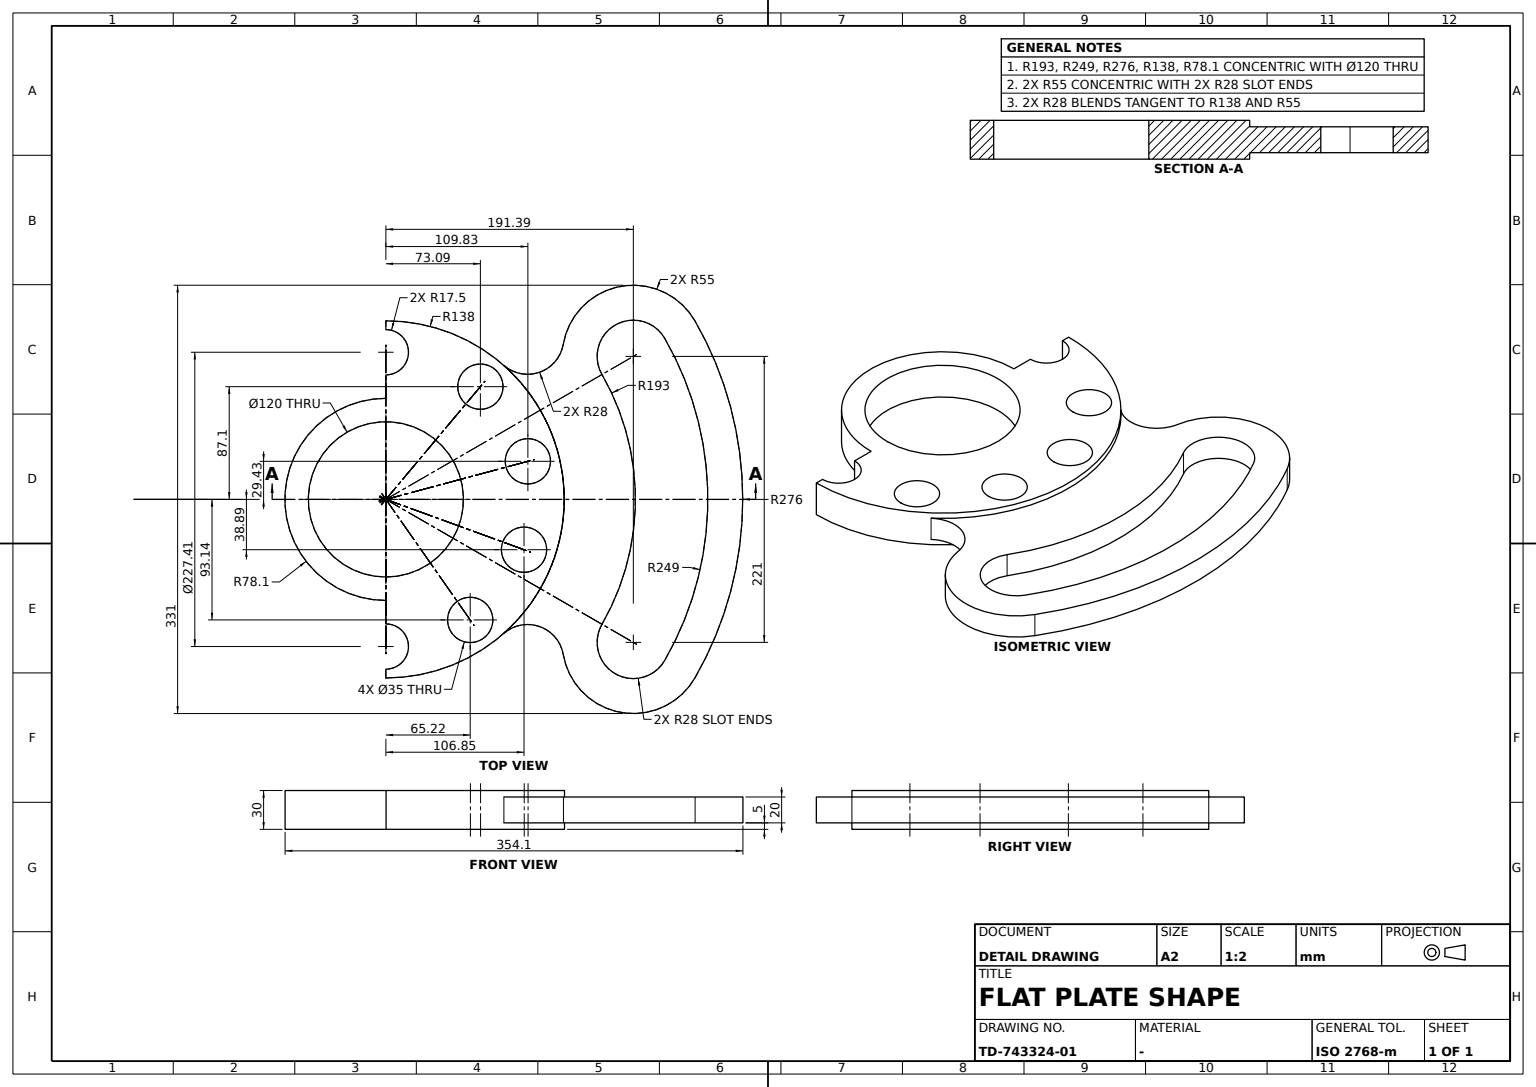
ISO-10303-21;
HEADER;
FILE_DESCRIPTION((''),'2;1');
FILE_NAME('','',(''),(''),'','','');
FILE_SCHEMA(('AUTOMOTIVE_DESIGN'));
ENDSEC;
DATA;
#1=APPLICATION_CONTEXT('');
#2=PRODUCT_CONTEXT('',#1,'mechanical');
#3=PRODUCT('','','',(#2));
#4=PRODUCT_DEFINITION_FORMATION('','',#3);
#5=PRODUCT_DEFINITION_CONTEXT('',#1,'design');
#6=PRODUCT_DEFINITION('','',#4,#5);
#7=PRODUCT_DEFINITION_SHAPE('','',#6);
#8=(LENGTH_UNIT()NAMED_UNIT(*)SI_UNIT(.MILLI.,.METRE.));
#9=(NAMED_UNIT(*)PLANE_ANGLE_UNIT()SI_UNIT($,.RADIAN.));
#10=(NAMED_UNIT(*)SI_UNIT($,.STERADIAN.)SOLID_ANGLE_UNIT());
#11=UNCERTAINTY_MEASURE_WITH_UNIT(LENGTH_MEASURE(0.005),#8,'distance_accuracy_value','');
#12=(GEOMETRIC_REPRESENTATION_CONTEXT(3)GLOBAL_UNCERTAINTY_ASSIGNED_CONTEXT((#11))GLOBAL_UNIT_ASSIGNED_CONTEXT((#8,#9,#10))REPRESENTATION_CONTEXT('',''));
#13=CARTESIAN_POINT('',(131.205128,0.,15.));
#14=VERTEX_POINT('',#13);
#15=CARTESIAN_POINT('',(138.,0.,15.));
#16=VERTEX_POINT('',#15);
#17=CARTESIAN_POINT('',(0.,0.,15.));
#18=DIRECTION('',(1.,0.,0.));
#19=VECTOR('',#18,1000.);
#20=LINE('',#17,#19);
#21=EDGE_CURVE('',#14,#16,#20,.T.);
#22=ORIENTED_EDGE('',*,*,#21,.F.);
#23=CARTESIAN_POINT('',(131.205128,0.,-15.));
#24=VERTEX_POINT('',#23);
#25=DIRECTION('',(0.,0.,1.));
#26=VECTOR('',#25,1000.);
#27=LINE('',#23,#26);
#28=EDGE_CURVE('',#24,#14,#27,.T.);
#29=ORIENTED_EDGE('',*,*,#28,.F.);
#30=CARTESIAN_POINT('',(138.,0.,-15.));
#31=VERTEX_POINT('',#30);
#32=CARTESIAN_POINT('',(0.,0.,-15.));
#33=LINE('',#32,#19);
#34=EDGE_CURVE('',#24,#31,#33,.T.);
#35=ORIENTED_EDGE('',*,*,#34,.T.);
#36=LINE('',#30,#26);
#37=EDGE_CURVE('',#31,#16,#36,.T.);
#38=ORIENTED_EDGE('',*,*,#37,.T.);
#39=EDGE_LOOP('',(#22,#29,#35,#38));
#40=FACE_BOUND('',#39,.T.);
#41=CARTESIAN_POINT('',(-138.,0.,0.));
#42=DIRECTION('',(0.,-1.,0.));
#43=AXIS2_PLACEMENT_3D('',#41,#42,#18);
#44=PLANE('',#43);
#45=ADVANCED_FACE('',(#40),#44,.T.);
#46=CARTESIAN_POINT('',(60.,0.,15.));
#47=VERTEX_POINT('',#46);
#48=AXIS2_PLACEMENT_3D('',#17,#25,#18);
#49=CIRCLE('',#48,60.);
#50=EDGE_CURVE('',#47,#47,#49,.T.);
#51=ORIENTED_EDGE('',*,*,#50,.T.);
#52=EDGE_LOOP('',(#51));
#53=FACE_BOUND('',#52,.T.);
#54=CARTESIAN_POINT('',(60.,0.,-15.));
#55=VERTEX_POINT('',#54);
#56=AXIS2_PLACEMENT_3D('',#32,#25,#18);
#57=CIRCLE('',#56,60.);
#58=EDGE_CURVE('',#55,#55,#57,.T.);
#59=ORIENTED_EDGE('',*,*,#58,.F.);
#60=EDGE_LOOP('',(#59));
#61=FACE_BOUND('',#60,.T.);
#62=CARTESIAN_POINT('',(0.,0.,9.34));
#63=AXIS2_PLACEMENT_3D('',#62,#25,#18);
#64=CYLINDRICAL_SURFACE('',#63,60.);
#65=ADVANCED_FACE('',(#53,#61),#64,.F.);
#66=CARTESIAN_POINT('',(56.389444,106.84787,15.));
#67=VERTEX_POINT('',#66);
#68=CARTESIAN_POINT('',(38.889444,106.84787,15.));
#69=AXIS2_PLACEMENT_3D('',#68,#25,#18);
#70=CIRCLE('',#69,17.5);
#71=EDGE_CURVE('',#67,#67,#70,.T.);
#72=ORIENTED_EDGE('',*,*,#71,.T.);
#73=EDGE_LOOP('',(#72));
#74=FACE_BOUND('',#73,.T.);
#75=CARTESIAN_POINT('',(56.389444,106.84787,-15.));
#76=VERTEX_POINT('',#75);
#77=CARTESIAN_POINT('',(38.889444,106.84787,-15.));
#78=AXIS2_PLACEMENT_3D('',#77,#25,#18);
#79=CIRCLE('',#78,17.5);
#80=EDGE_CURVE('',#76,#76,#79,.T.);
#81=ORIENTED_EDGE('',*,*,#80,.F.);
#82=EDGE_LOOP('',(#81));
#83=FACE_BOUND('',#82,.T.);
#84=CARTESIAN_POINT('',(38.889444,106.84787,9.34));
#85=AXIS2_PLACEMENT_3D('',#84,#25,#18);
#86=CYLINDRICAL_SURFACE('',#85,17.5);
#87=ADVANCED_FACE('',(#74,#83),#86,.F.);
#88=CARTESIAN_POINT('',(-78.102497,0.,-15.));
#89=VERTEX_POINT('',#88);
#90=CARTESIAN_POINT('',(-78.102497,0.,15.));
#91=VERTEX_POINT('',#90);
#92=LINE('',#88,#26);
#93=EDGE_CURVE('',#89,#91,#92,.T.);
#94=ORIENTED_EDGE('',*,*,#93,.F.);
#95=CARTESIAN_POINT('',(78.102497,0.,-15.));
#96=VERTEX_POINT('',#95);
#97=CIRCLE('',#56,78.102497);
#98=EDGE_CURVE('',#89,#96,#97,.T.);
#99=ORIENTED_EDGE('',*,*,#98,.T.);
#100=CARTESIAN_POINT('',(78.102497,0.,15.));
#101=VERTEX_POINT('',#100);
#102=LINE('',#95,#26);
#103=EDGE_CURVE('',#96,#101,#102,.T.);
#104=ORIENTED_EDGE('',*,*,#103,.T.);
#105=CIRCLE('',#48,78.102497);
#106=EDGE_CURVE('',#91,#101,#105,.T.);
#107=ORIENTED_EDGE('',*,*,#106,.F.);
#108=EDGE_LOOP('',(#94,#99,#104,#107));
#109=FACE_BOUND('',#108,.T.);
#110=CARTESIAN_POINT('',(0.,0.,0.));
#111=AXIS2_PLACEMENT_3D('',#110,#25,#18);
#112=CYLINDRICAL_SURFACE('',#111,78.102497);
#113=ADVANCED_FACE('',(#109),#112,.T.);
#114=CARTESIAN_POINT('',(96.205128,0.,15.));
#115=VERTEX_POINT('',#114);
#116=CARTESIAN_POINT('',(96.205128,0.,-15.));
#117=VERTEX_POINT('',#116);
#118=LINE('',#116,#26);
#119=EDGE_CURVE('',#115,#117,#118,.F.);
#120=ORIENTED_EDGE('',*,*,#119,.F.);
#121=EDGE_CURVE('',#101,#115,#20,.T.);
#122=ORIENTED_EDGE('',*,*,#121,.F.);
#123=ORIENTED_EDGE('',*,*,#103,.F.);
#124=EDGE_CURVE('',#96,#117,#33,.T.);
#125=ORIENTED_EDGE('',*,*,#124,.T.);
#126=EDGE_LOOP('',(#120,#122,#123,#125));
#127=FACE_BOUND('',#126,.T.);
#128=ADVANCED_FACE('',(#127),#44,.T.);
#129=CARTESIAN_POINT('',(124.5,215.640326,10.));
#130=VERTEX_POINT('',#129);
#131=CARTESIAN_POINT('',(-124.5,215.640326,10.));
#132=VERTEX_POINT('',#131);
#133=CARTESIAN_POINT('',(0.,0.,10.));
#134=AXIS2_PLACEMENT_3D('',#133,#25,#18);
#135=CIRCLE('',#134,249.);
#136=EDGE_CURVE('',#130,#132,#135,.T.);
#137=ORIENTED_EDGE('',*,*,#136,.T.);
#138=CARTESIAN_POINT('',(-124.5,215.640326,-10.));
#139=VERTEX_POINT('',#138);
#140=CARTESIAN_POINT('',(-124.5,215.640326,0.));
#141=LINE('',#140,#26);
#142=EDGE_CURVE('',#132,#139,#141,.F.);
#143=ORIENTED_EDGE('',*,*,#142,.T.);
#144=CARTESIAN_POINT('',(124.5,215.640326,-10.));
#145=VERTEX_POINT('',#144);
#146=CARTESIAN_POINT('',(0.,0.,-10.));
#147=AXIS2_PLACEMENT_3D('',#146,#25,#18);
#148=CIRCLE('',#147,249.);
#149=EDGE_CURVE('',#145,#139,#148,.T.);
#150=ORIENTED_EDGE('',*,*,#149,.F.);
#151=CARTESIAN_POINT('',(124.5,215.640326,0.));
#152=LINE('',#151,#26);
#153=EDGE_CURVE('',#130,#145,#152,.F.);
#154=ORIENTED_EDGE('',*,*,#153,.F.);
#155=EDGE_LOOP('',(#137,#143,#150,#154));
#156=FACE_BOUND('',#155,.T.);
#157=CYLINDRICAL_SURFACE('',#63,249.);
#158=ADVANCED_FACE('',(#156),#157,.F.);
#159=CARTESIAN_POINT('',(-119.887477,137.198669,-10.));
#160=VERTEX_POINT('',#159);
#161=CARTESIAN_POINT('',(-119.887477,137.198669,10.));
#162=VERTEX_POINT('',#161);
#163=CARTESIAN_POINT('',(-119.887477,137.198669,0.));
#164=LINE('',#163,#26);
#165=EDGE_CURVE('',#160,#162,#164,.T.);
#166=ORIENTED_EDGE('',*,*,#165,.F.);
#167=CARTESIAN_POINT('',(-103.638462,91.121179,-10.));
#168=VERTEX_POINT('',#167);
#169=CARTESIAN_POINT('',(-124.666556,109.609534,-10.));
#170=AXIS2_PLACEMENT_3D('',#169,#25,#18);
#171=CIRCLE('',#170,28.);
#172=EDGE_CURVE('',#168,#160,#171,.T.);
#173=ORIENTED_EDGE('',*,*,#172,.F.);
#174=CARTESIAN_POINT('',(-103.638462,91.121179,10.));
#175=VERTEX_POINT('',#174);
#176=CARTESIAN_POINT('',(-103.638462,91.121179,0.));
#177=LINE('',#176,#26);
#178=EDGE_CURVE('',#168,#175,#177,.T.);
#179=ORIENTED_EDGE('',*,*,#178,.T.);
#180=CARTESIAN_POINT('',(-124.666556,109.609534,10.));
#181=AXIS2_PLACEMENT_3D('',#180,#25,#18);
#182=CIRCLE('',#181,28.);
#183=EDGE_CURVE('',#175,#162,#182,.T.);
#184=ORIENTED_EDGE('',*,*,#183,.T.);
#185=EDGE_LOOP('',(#166,#173,#179,#184));
#186=FACE_BOUND('',#185,.T.);
#187=CARTESIAN_POINT('',(-124.666556,109.609534,0.));
#188=AXIS2_PLACEMENT_3D('',#187,#25,#18);
#189=CYLINDRICAL_SURFACE('',#188,28.);
#190=ADVANCED_FACE('',(#186),#189,.F.);
#191=CARTESIAN_POINT('',(96.5,167.142903,10.));
#192=VERTEX_POINT('',#191);
#193=CARTESIAN_POINT('',(110.5,191.391614,10.));
#194=AXIS2_PLACEMENT_3D('',#193,#25,#18);
#195=CIRCLE('',#194,28.);
#196=EDGE_CURVE('',#192,#130,#195,.T.);
#197=ORIENTED_EDGE('',*,*,#196,.T.);
#198=ORIENTED_EDGE('',*,*,#153,.T.);
#199=CARTESIAN_POINT('',(96.5,167.142903,-10.));
#200=VERTEX_POINT('',#199);
#201=CARTESIAN_POINT('',(110.5,191.391614,-10.));
#202=AXIS2_PLACEMENT_3D('',#201,#25,#18);
#203=CIRCLE('',#202,28.);
#204=EDGE_CURVE('',#200,#145,#203,.T.);
#205=ORIENTED_EDGE('',*,*,#204,.F.);
#206=CARTESIAN_POINT('',(96.5,167.142903,0.));
#207=LINE('',#206,#26);
#208=EDGE_CURVE('',#192,#200,#207,.F.);
#209=ORIENTED_EDGE('',*,*,#208,.F.);
#210=EDGE_LOOP('',(#197,#198,#205,#209));
#211=FACE_BOUND('',#210,.T.);
#212=CARTESIAN_POINT('',(110.5,191.391614,9.34));
#213=AXIS2_PLACEMENT_3D('',#212,#25,#18);
#214=CYLINDRICAL_SURFACE('',#213,28.);
#215=ADVANCED_FACE('',(#211),#214,.F.);
#216=CARTESIAN_POINT('',(138.,239.023011,-10.));
#217=VERTEX_POINT('',#216);
#218=CARTESIAN_POINT('',(138.,239.023011,10.));
#219=VERTEX_POINT('',#218);
#220=CARTESIAN_POINT('',(138.,239.023011,0.));
#221=LINE('',#220,#26);
#222=EDGE_CURVE('',#217,#219,#221,.T.);
#223=ORIENTED_EDGE('',*,*,#222,.T.);
#224=CARTESIAN_POINT('',(119.887477,137.198669,10.));
#225=VERTEX_POINT('',#224);
#226=CIRCLE('',#194,55.);
#227=EDGE_CURVE('',#225,#219,#226,.T.);
#228=ORIENTED_EDGE('',*,*,#227,.F.);
#229=CARTESIAN_POINT('',(119.887477,137.198669,-10.));
#230=VERTEX_POINT('',#229);
#231=CARTESIAN_POINT('',(119.887477,137.198669,0.));
#232=LINE('',#231,#26);
#233=EDGE_CURVE('',#230,#225,#232,.T.);
#234=ORIENTED_EDGE('',*,*,#233,.F.);
#235=CIRCLE('',#202,55.);
#236=EDGE_CURVE('',#230,#217,#235,.T.);
#237=ORIENTED_EDGE('',*,*,#236,.T.);
#238=EDGE_LOOP('',(#223,#228,#234,#237));
#239=FACE_BOUND('',#238,.T.);
#240=CARTESIAN_POINT('',(110.5,191.391614,0.));
#241=AXIS2_PLACEMENT_3D('',#240,#25,#18);
#242=CYLINDRICAL_SURFACE('',#241,55.);
#243=ADVANCED_FACE('',(#239),#242,.T.);
#244=CARTESIAN_POINT('',(-11.929053,109.83072,-15.));
#245=VERTEX_POINT('',#244);
#246=CARTESIAN_POINT('',(-29.429053,109.83072,-15.));
#247=AXIS2_PLACEMENT_3D('',#246,#25,#18);
#248=CIRCLE('',#247,17.5);
#249=EDGE_CURVE('',#245,#245,#248,.T.);
#250=ORIENTED_EDGE('',*,*,#249,.F.);
#251=EDGE_LOOP('',(#250));
#252=FACE_BOUND('',#251,.T.);
#253=CARTESIAN_POINT('',(-11.929053,109.83072,15.));
#254=VERTEX_POINT('',#253);
#255=CARTESIAN_POINT('',(-29.429053,109.83072,15.));
#256=AXIS2_PLACEMENT_3D('',#255,#25,#18);
#257=CIRCLE('',#256,17.5);
#258=EDGE_CURVE('',#254,#254,#257,.T.);
#259=ORIENTED_EDGE('',*,*,#258,.T.);
#260=EDGE_LOOP('',(#259));
#261=FACE_BOUND('',#260,.T.);
#262=CARTESIAN_POINT('',(-29.429053,109.83072,9.34));
#263=AXIS2_PLACEMENT_3D('',#262,#25,#18);
#264=CYLINDRICAL_SURFACE('',#263,17.5);
#265=ADVANCED_FACE('',(#252,#261),#264,.F.);
#266=CARTESIAN_POINT('',(-131.205128,0.,-15.));
#267=VERTEX_POINT('',#266);
#268=CARTESIAN_POINT('',(-131.205128,0.,15.));
#269=VERTEX_POINT('',#268);
#270=LINE('',#268,#26);
#271=EDGE_CURVE('',#267,#269,#270,.T.);
#272=ORIENTED_EDGE('',*,*,#271,.F.);
#273=CARTESIAN_POINT('',(-96.205128,0.,-15.));
#274=VERTEX_POINT('',#273);
#275=CARTESIAN_POINT('',(-113.705128,0.,-15.));
#276=AXIS2_PLACEMENT_3D('',#275,#25,#18);
#277=CIRCLE('',#276,17.5);
#278=EDGE_CURVE('',#274,#267,#277,.T.);
#279=ORIENTED_EDGE('',*,*,#278,.F.);
#280=CARTESIAN_POINT('',(-96.205128,0.,15.));
#281=VERTEX_POINT('',#280);
#282=LINE('',#280,#26);
#283=EDGE_CURVE('',#281,#274,#282,.F.);
#284=ORIENTED_EDGE('',*,*,#283,.F.);
#285=CARTESIAN_POINT('',(-113.705128,0.,15.));
#286=AXIS2_PLACEMENT_3D('',#285,#25,#18);
#287=CIRCLE('',#286,17.5);
#288=EDGE_CURVE('',#281,#269,#287,.T.);
#289=ORIENTED_EDGE('',*,*,#288,.T.);
#290=EDGE_LOOP('',(#272,#279,#284,#289));
#291=FACE_BOUND('',#290,.T.);
#292=CARTESIAN_POINT('',(-113.705128,0.,9.34));
#293=AXIS2_PLACEMENT_3D('',#292,#25,#18);
#294=CYLINDRICAL_SURFACE('',#293,17.5);
#295=ADVANCED_FACE('',(#291),#294,.F.);
#296=CARTESIAN_POINT('',(-138.,239.023011,-10.));
#297=VERTEX_POINT('',#296);
#298=CARTESIAN_POINT('',(-138.,239.023011,10.));
#299=VERTEX_POINT('',#298);
#300=CARTESIAN_POINT('',(-138.,239.023011,0.));
#301=LINE('',#300,#26);
#302=EDGE_CURVE('',#297,#299,#301,.T.);
#303=ORIENTED_EDGE('',*,*,#302,.F.);
#304=CARTESIAN_POINT('',(-110.5,191.391614,-10.));
#305=AXIS2_PLACEMENT_3D('',#304,#25,#18);
#306=CIRCLE('',#305,55.);
#307=EDGE_CURVE('',#297,#160,#306,.T.);
#308=ORIENTED_EDGE('',*,*,#307,.T.);
#309=ORIENTED_EDGE('',*,*,#165,.T.);
#310=CARTESIAN_POINT('',(-110.5,191.391614,10.));
#311=AXIS2_PLACEMENT_3D('',#310,#25,#18);
#312=CIRCLE('',#311,55.);
#313=EDGE_CURVE('',#299,#162,#312,.T.);
#314=ORIENTED_EDGE('',*,*,#313,.F.);
#315=EDGE_LOOP('',(#303,#308,#309,#314));
#316=FACE_BOUND('',#315,.T.);
#317=CARTESIAN_POINT('',(-110.5,191.391614,0.));
#318=AXIS2_PLACEMENT_3D('',#317,#25,#18);
#319=CYLINDRICAL_SURFACE('',#318,55.);
#320=ADVANCED_FACE('',(#316),#319,.T.);
#321=ORIENTED_EDGE('',*,*,#302,.T.);
#322=CIRCLE('',#134,276.);
#323=EDGE_CURVE('',#219,#299,#322,.T.);
#324=ORIENTED_EDGE('',*,*,#323,.F.);
#325=ORIENTED_EDGE('',*,*,#222,.F.);
#326=CIRCLE('',#147,276.);
#327=EDGE_CURVE('',#217,#297,#326,.T.);
#328=ORIENTED_EDGE('',*,*,#327,.T.);
#329=EDGE_LOOP('',(#321,#324,#325,#328));
#330=FACE_BOUND('',#329,.T.);
#331=CYLINDRICAL_SURFACE('',#111,276.);
#332=ADVANCED_FACE('',(#330),#331,.T.);
#333=CARTESIAN_POINT('',(-69.603181,73.088247,-15.));
#334=VERTEX_POINT('',#333);
#335=CARTESIAN_POINT('',(-87.103181,73.088247,-15.));
#336=AXIS2_PLACEMENT_3D('',#335,#25,#18);
#337=CIRCLE('',#336,17.5);
#338=EDGE_CURVE('',#334,#334,#337,.T.);
#339=ORIENTED_EDGE('',*,*,#338,.F.);
#340=EDGE_LOOP('',(#339));
#341=FACE_BOUND('',#340,.T.);
#342=CARTESIAN_POINT('',(-69.603181,73.088247,15.));
#343=VERTEX_POINT('',#342);
#344=CARTESIAN_POINT('',(-87.103181,73.088247,15.));
#345=AXIS2_PLACEMENT_3D('',#344,#25,#18);
#346=CIRCLE('',#345,17.5);
#347=EDGE_CURVE('',#343,#343,#346,.T.);
#348=ORIENTED_EDGE('',*,*,#347,.T.);
#349=EDGE_LOOP('',(#348));
#350=FACE_BOUND('',#349,.T.);
#351=CARTESIAN_POINT('',(-87.103181,73.088247,9.34));
#352=AXIS2_PLACEMENT_3D('',#351,#25,#18);
#353=CYLINDRICAL_SURFACE('',#352,17.5);
#354=ADVANCED_FACE('',(#341,#350),#353,.F.);
#355=CARTESIAN_POINT('',(-96.5,167.142903,10.));
#356=VERTEX_POINT('',#355);
#357=CIRCLE('',#134,193.);
#358=EDGE_CURVE('',#192,#356,#357,.T.);
#359=ORIENTED_EDGE('',*,*,#358,.F.);
#360=ORIENTED_EDGE('',*,*,#208,.T.);
#361=CARTESIAN_POINT('',(-96.5,167.142903,-10.));
#362=VERTEX_POINT('',#361);
#363=CIRCLE('',#147,193.);
#364=EDGE_CURVE('',#200,#362,#363,.T.);
#365=ORIENTED_EDGE('',*,*,#364,.T.);
#366=CARTESIAN_POINT('',(-96.5,167.142903,0.));
#367=LINE('',#366,#26);
#368=EDGE_CURVE('',#356,#362,#367,.F.);
#369=ORIENTED_EDGE('',*,*,#368,.F.);
#370=EDGE_LOOP('',(#359,#360,#365,#369));
#371=FACE_BOUND('',#370,.T.);
#372=CYLINDRICAL_SURFACE('',#63,193.);
#373=ADVANCED_FACE('',(#371),#372,.T.);
#374=CARTESIAN_POINT('',(113.705128,0.,-15.));
#375=AXIS2_PLACEMENT_3D('',#374,#25,#18);
#376=CIRCLE('',#375,17.5);
#377=EDGE_CURVE('',#24,#117,#376,.T.);
#378=ORIENTED_EDGE('',*,*,#377,.F.);
#379=ORIENTED_EDGE('',*,*,#28,.T.);
#380=CARTESIAN_POINT('',(113.705128,0.,15.));
#381=AXIS2_PLACEMENT_3D('',#380,#25,#18);
#382=CIRCLE('',#381,17.5);
#383=EDGE_CURVE('',#14,#115,#382,.T.);
#384=ORIENTED_EDGE('',*,*,#383,.T.);
#385=ORIENTED_EDGE('',*,*,#119,.T.);
#386=EDGE_LOOP('',(#378,#379,#384,#385));
#387=FACE_BOUND('',#386,.T.);
#388=CARTESIAN_POINT('',(113.705128,0.,9.34));
#389=AXIS2_PLACEMENT_3D('',#388,#25,#18);
#390=CYLINDRICAL_SURFACE('',#389,17.5);
#391=ADVANCED_FACE('',(#387),#390,.F.);
#392=ORIENTED_EDGE('',*,*,#71,.F.);
#393=EDGE_LOOP('',(#392));
#394=FACE_BOUND('',#393,.T.);
#395=ORIENTED_EDGE('',*,*,#258,.F.);
#396=EDGE_LOOP('',(#395));
#397=FACE_BOUND('',#396,.T.);
#398=ORIENTED_EDGE('',*,*,#50,.F.);
#399=EDGE_LOOP('',(#398));
#400=FACE_BOUND('',#399,.T.);
#401=CARTESIAN_POINT('',(110.641788,65.218582,15.));
#402=VERTEX_POINT('',#401);
#403=CARTESIAN_POINT('',(93.141788,65.218582,15.));
#404=AXIS2_PLACEMENT_3D('',#403,#25,#18);
#405=CIRCLE('',#404,17.5);
#406=EDGE_CURVE('',#402,#402,#405,.T.);
#407=ORIENTED_EDGE('',*,*,#406,.F.);
#408=EDGE_LOOP('',(#407));
#409=FACE_BOUND('',#408,.T.);
#410=ORIENTED_EDGE('',*,*,#288,.F.);
#411=EDGE_CURVE('',#281,#91,#20,.T.);
#412=ORIENTED_EDGE('',*,*,#411,.T.);
#413=ORIENTED_EDGE('',*,*,#106,.T.);
#414=ORIENTED_EDGE('',*,*,#121,.T.);
#415=ORIENTED_EDGE('',*,*,#383,.F.);
#416=ORIENTED_EDGE('',*,*,#21,.T.);
#417=CARTESIAN_POINT('',(-138.,0.,15.));
#418=VERTEX_POINT('',#417);
#419=CIRCLE('',#48,138.);
#420=EDGE_CURVE('',#16,#418,#419,.T.);
#421=ORIENTED_EDGE('',*,*,#420,.T.);
#422=EDGE_CURVE('',#418,#269,#20,.T.);
#423=ORIENTED_EDGE('',*,*,#422,.T.);
#424=EDGE_LOOP('',(#410,#412,#413,#414,#415,#416,#421,#423));
#425=FACE_BOUND('',#424,.T.);
#426=ORIENTED_EDGE('',*,*,#347,.F.);
#427=EDGE_LOOP('',(#426));
#428=FACE_BOUND('',#427,.T.);
#429=PLANE('',#48);
#430=ADVANCED_FACE('',(#394,#397,#400,#409,#425,#428),#429,.T.);
#431=CIRCLE('',#305,28.);
#432=EDGE_CURVE('',#139,#362,#431,.T.);
#433=ORIENTED_EDGE('',*,*,#432,.T.);
#434=ORIENTED_EDGE('',*,*,#364,.F.);
#435=ORIENTED_EDGE('',*,*,#204,.T.);
#436=ORIENTED_EDGE('',*,*,#149,.T.);
#437=EDGE_LOOP('',(#433,#434,#435,#436));
#438=FACE_BOUND('',#437,.T.);
#439=CARTESIAN_POINT('',(103.638462,91.121179,-10.));
#440=VERTEX_POINT('',#439);
#441=CARTESIAN_POINT('',(124.666556,109.609534,-10.));
#442=AXIS2_PLACEMENT_3D('',#441,#25,#18);
#443=CIRCLE('',#442,28.);
#444=EDGE_CURVE('',#230,#440,#443,.T.);
#445=ORIENTED_EDGE('',*,*,#444,.T.);
#446=CIRCLE('',#147,138.);
#447=EDGE_CURVE('',#440,#168,#446,.T.);
#448=ORIENTED_EDGE('',*,*,#447,.T.);
#449=ORIENTED_EDGE('',*,*,#172,.T.);
#450=ORIENTED_EDGE('',*,*,#307,.F.);
#451=ORIENTED_EDGE('',*,*,#327,.F.);
#452=ORIENTED_EDGE('',*,*,#236,.F.);
#453=EDGE_LOOP('',(#445,#448,#449,#450,#451,#452));
#454=FACE_BOUND('',#453,.T.);
#455=PLANE('',#147);
#456=ADVANCED_FACE('',(#438,#454),#455,.F.);
#457=CARTESIAN_POINT('',(103.638462,91.121179,10.));
#458=VERTEX_POINT('',#457);
#459=CIRCLE('',#134,138.);
#460=EDGE_CURVE('',#458,#175,#459,.T.);
#461=ORIENTED_EDGE('',*,*,#460,.F.);
#462=CARTESIAN_POINT('',(124.666556,109.609534,10.));
#463=AXIS2_PLACEMENT_3D('',#462,#25,#18);
#464=CIRCLE('',#463,28.);
#465=EDGE_CURVE('',#225,#458,#464,.T.);
#466=ORIENTED_EDGE('',*,*,#465,.F.);
#467=ORIENTED_EDGE('',*,*,#227,.T.);
#468=ORIENTED_EDGE('',*,*,#323,.T.);
#469=ORIENTED_EDGE('',*,*,#313,.T.);
#470=ORIENTED_EDGE('',*,*,#183,.F.);
#471=EDGE_LOOP('',(#461,#466,#467,#468,#469,#470));
#472=FACE_BOUND('',#471,.T.);
#473=ORIENTED_EDGE('',*,*,#136,.F.);
#474=ORIENTED_EDGE('',*,*,#196,.F.);
#475=ORIENTED_EDGE('',*,*,#358,.T.);
#476=CIRCLE('',#311,28.);
#477=EDGE_CURVE('',#132,#356,#476,.T.);
#478=ORIENTED_EDGE('',*,*,#477,.F.);
#479=EDGE_LOOP('',(#473,#474,#475,#478));
#480=FACE_BOUND('',#479,.T.);
#481=PLANE('',#134);
#482=ADVANCED_FACE('',(#472,#480),#481,.T.);
#483=CARTESIAN_POINT('',(110.641788,65.218582,-15.));
#484=VERTEX_POINT('',#483);
#485=CARTESIAN_POINT('',(93.141788,65.218582,-15.));
#486=AXIS2_PLACEMENT_3D('',#485,#25,#18);
#487=CIRCLE('',#486,17.5);
#488=EDGE_CURVE('',#484,#484,#487,.T.);
#489=ORIENTED_EDGE('',*,*,#488,.F.);
#490=EDGE_LOOP('',(#489));
#491=FACE_BOUND('',#490,.T.);
#492=ORIENTED_EDGE('',*,*,#406,.T.);
#493=EDGE_LOOP('',(#492));
#494=FACE_BOUND('',#493,.T.);
#495=CARTESIAN_POINT('',(93.141788,65.218582,9.34));
#496=AXIS2_PLACEMENT_3D('',#495,#25,#18);
#497=CYLINDRICAL_SURFACE('',#496,17.5);
#498=ADVANCED_FACE('',(#491,#494),#497,.F.);
#499=ORIENTED_EDGE('',*,*,#124,.F.);
#500=ORIENTED_EDGE('',*,*,#98,.F.);
#501=EDGE_CURVE('',#274,#89,#33,.T.);
#502=ORIENTED_EDGE('',*,*,#501,.F.);
#503=ORIENTED_EDGE('',*,*,#278,.T.);
#504=CARTESIAN_POINT('',(-138.,0.,-15.));
#505=VERTEX_POINT('',#504);
#506=EDGE_CURVE('',#505,#267,#33,.T.);
#507=ORIENTED_EDGE('',*,*,#506,.F.);
#508=CIRCLE('',#56,138.);
#509=EDGE_CURVE('',#31,#505,#508,.T.);
#510=ORIENTED_EDGE('',*,*,#509,.F.);
#511=ORIENTED_EDGE('',*,*,#34,.F.);
#512=ORIENTED_EDGE('',*,*,#377,.T.);
#513=EDGE_LOOP('',(#499,#500,#502,#503,#507,#510,#511,#512));
#514=FACE_BOUND('',#513,.T.);
#515=ORIENTED_EDGE('',*,*,#488,.T.);
#516=EDGE_LOOP('',(#515));
#517=FACE_BOUND('',#516,.T.);
#518=ORIENTED_EDGE('',*,*,#338,.T.);
#519=EDGE_LOOP('',(#518));
#520=FACE_BOUND('',#519,.T.);
#521=ORIENTED_EDGE('',*,*,#249,.T.);
#522=EDGE_LOOP('',(#521));
#523=FACE_BOUND('',#522,.T.);
#524=ORIENTED_EDGE('',*,*,#58,.T.);
#525=EDGE_LOOP('',(#524));
#526=FACE_BOUND('',#525,.T.);
#527=ORIENTED_EDGE('',*,*,#80,.T.);
#528=EDGE_LOOP('',(#527));
#529=FACE_BOUND('',#528,.T.);
#530=PLANE('',#56);
#531=ADVANCED_FACE('',(#514,#517,#520,#523,#526,#529),#530,.F.);
#532=ORIENTED_EDGE('',*,*,#142,.F.);
#533=ORIENTED_EDGE('',*,*,#477,.T.);
#534=ORIENTED_EDGE('',*,*,#368,.T.);
#535=ORIENTED_EDGE('',*,*,#432,.F.);
#536=EDGE_LOOP('',(#532,#533,#534,#535));
#537=FACE_BOUND('',#536,.T.);
#538=CARTESIAN_POINT('',(-110.5,191.391614,9.34));
#539=AXIS2_PLACEMENT_3D('',#538,#25,#18);
#540=CYLINDRICAL_SURFACE('',#539,28.);
#541=ADVANCED_FACE('',(#537),#540,.F.);
#542=ORIENTED_EDGE('',*,*,#93,.T.);
#543=ORIENTED_EDGE('',*,*,#411,.F.);
#544=ORIENTED_EDGE('',*,*,#283,.T.);
#545=ORIENTED_EDGE('',*,*,#501,.T.);
#546=EDGE_LOOP('',(#542,#543,#544,#545));
#547=FACE_BOUND('',#546,.T.);
#548=ADVANCED_FACE('',(#547),#44,.T.);
#549=ORIENTED_EDGE('',*,*,#506,.T.);
#550=ORIENTED_EDGE('',*,*,#271,.T.);
#551=ORIENTED_EDGE('',*,*,#422,.F.);
#552=LINE('',#504,#26);
#553=EDGE_CURVE('',#505,#418,#552,.T.);
#554=ORIENTED_EDGE('',*,*,#553,.F.);
#555=EDGE_LOOP('',(#549,#550,#551,#554));
#556=FACE_BOUND('',#555,.T.);
#557=ADVANCED_FACE('',(#556),#44,.T.);
#558=ORIENTED_EDGE('',*,*,#178,.F.);
#559=ORIENTED_EDGE('',*,*,#447,.F.);
#560=CARTESIAN_POINT('',(103.638462,91.121179,0.));
#561=LINE('',#560,#26);
#562=EDGE_CURVE('',#440,#458,#561,.T.);
#563=ORIENTED_EDGE('',*,*,#562,.T.);
#564=ORIENTED_EDGE('',*,*,#460,.T.);
#565=EDGE_LOOP('',(#558,#559,#563,#564));
#566=FACE_BOUND('',#565,.T.);
#567=ORIENTED_EDGE('',*,*,#37,.F.);
#568=ORIENTED_EDGE('',*,*,#509,.T.);
#569=ORIENTED_EDGE('',*,*,#553,.T.);
#570=ORIENTED_EDGE('',*,*,#420,.F.);
#571=EDGE_LOOP('',(#567,#568,#569,#570));
#572=FACE_BOUND('',#571,.T.);
#573=CYLINDRICAL_SURFACE('',#111,138.);
#574=ADVANCED_FACE('',(#566,#572),#573,.T.);
#575=ORIENTED_EDGE('',*,*,#465,.T.);
#576=ORIENTED_EDGE('',*,*,#562,.F.);
#577=ORIENTED_EDGE('',*,*,#444,.F.);
#578=ORIENTED_EDGE('',*,*,#233,.T.);
#579=EDGE_LOOP('',(#575,#576,#577,#578));
#580=FACE_BOUND('',#579,.T.);
#581=CARTESIAN_POINT('',(124.666556,109.609534,0.));
#582=AXIS2_PLACEMENT_3D('',#581,#25,#18);
#583=CYLINDRICAL_SURFACE('',#582,28.);
#584=ADVANCED_FACE('',(#580),#583,.F.);
#585=CLOSED_SHELL('',(#45,#65,#87,#113,#128,#158,#190,#215,#243,#265,#295,#320,#332,#354,#373,#391,#430,#456,#482,#498,#531,#541,#548,#557,#574,#584));
#586=MANIFOLD_SOLID_BREP('',#585);
#587=ADVANCED_BREP_SHAPE_REPRESENTATION('',(#586),#12);
#588=SHAPE_DEFINITION_REPRESENTATION(#7,#587);
ENDSEC;
END-ISO-10303-21;
